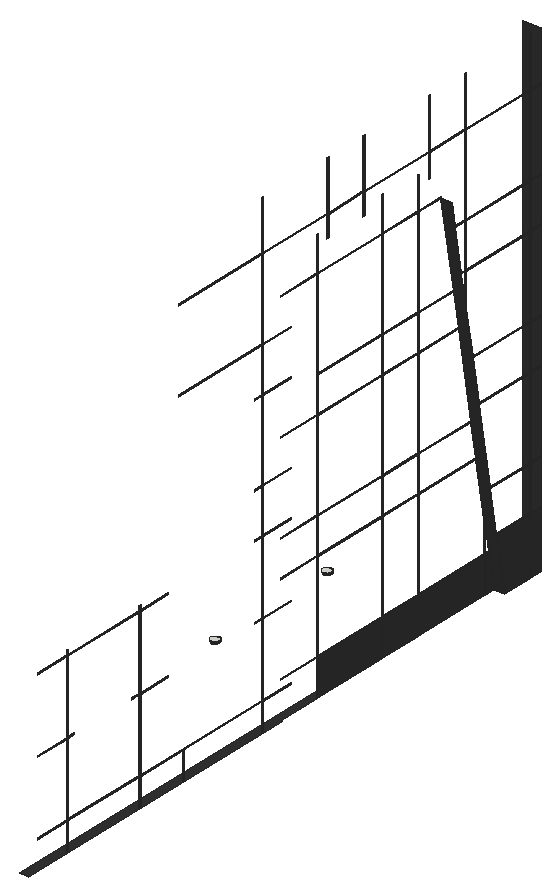
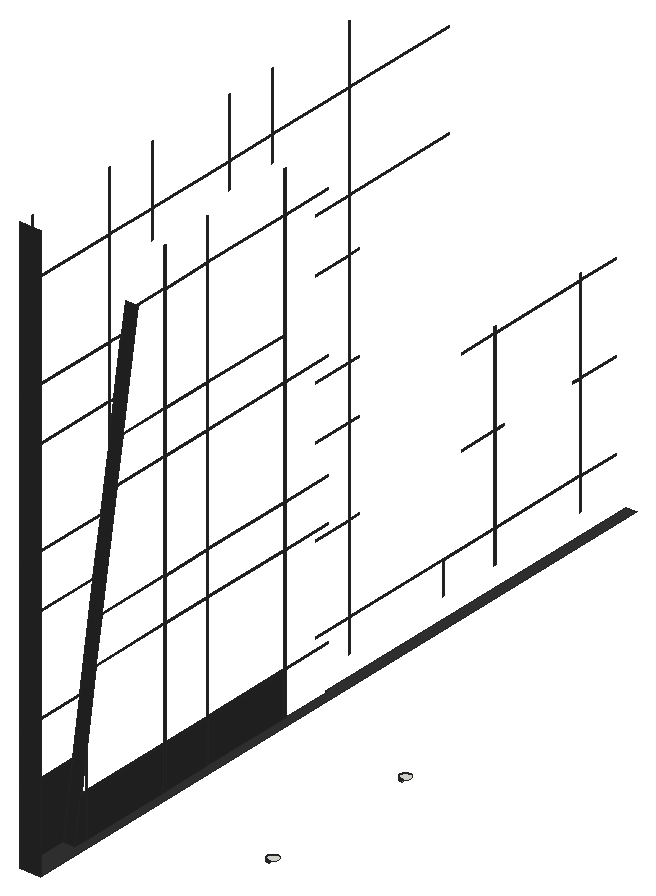
# SketchUp Ruby script. Lengths in inches.
U = 1.inch
M = Sketchup.active_model
def pt(a) = Geom::Point3d.new(a.map { |v| v * U })
def face(e, loops, mat)
  f = e.add_face(loops[0].map { |a| pt(a) })
  loops[1..].each { |l| e.add_face(l.map { |a| pt(a) }).erase! }
  f.material = f.back_material = mat if mat
  f
end
# faces: each face lists its corners as indices into pts; further lists are holes
def faces(e, pts, list, mat = nil) = list.each { |f| face(e, (f[0].is_a?(Array) ? f : [f]).map { |l| l.map { |i| pts[i] } }, mat) }
# xy, xz, yz: faces in a plane at the given z, y or x. An outline is a flat list of corners, or four numbers for a rectangle; further outlines are holes
def ring(l) = l.size == 4 ? [[l[0], l[1]], [l[2], l[1]], [l[2], l[3]], [l[0], l[3]]] : l.each_slice(2).to_a
def flat(e, list, mat, &to3) = list.each { |f| face(e, (f[0].is_a?(Array) ? f : [f]).map { |l| ring(l).map { |u, v| to3.(u, v) } }, mat) }
def xy(e, z, list, mat = nil) = flat(e, list, mat) { |x, y| [x, y, z] }
def xz(e, y, list, mat = nil) = flat(e, list, mat) { |x, z| [x, y, z] }
def yz(e, x, list, mat = nil) = flat(e, list, mat) { |y, z| [x, y, z] }
def lines(e, pts, list) = list.each { |a, b| e.add_line(pt(pts[a]), pt(pts[b])) }
# prism: a flat outline (further loops are holes) pulled along v
def prism(e, loops, v, mat = nil)
  f = face(e, loops, mat); d = Geom::Vector3d.new(v.map { |x| x * U })
  f.pushpull(f.normal.samedirection?(d) ? d.length : -d.length)
end
def box(e, o, s, mat = nil) = prism(e, [[o, [o[0] + s[0], o[1], o[2]], [o[0] + s[0], o[1] + s[1], o[2]], [o[0], o[1] + s[1], o[2]]]], [0, 0, s[2]], mat)
def at(x, y, z, deg = 0) = Geom::Transformation.translation(pt([x, y, z])) * Geom::Transformation.rotation(ORIGIN, Z_AXIS, deg.degrees)
def axes(o, x, y, z) = Geom::Transformation.new([*x, 0, *y, 0, *z, 0, *pt(o).to_a, 1])
def part(name) = M.definitions.add(name)
# library, detail: a bought-in or finely detailed component or shape, given as its bounding box
def library(name, o, s) = part(name).tap { |d| box(d.entities, o, s) }
def detail(e, o, s) = box(e.add_group.entities, o, s)
def put(e, d, t, mat = nil) = e.add_instance(d, t).tap { |i| i.material = mat if mat }
def group(e, t, mat = nil) = e.add_group.tap { |g| g.transformation = t; g.material = mat if mat }.entities
root = M.entities
M.materials.add("[Granite Dark Gray]").color = [51, 50, 50]
xy(root,126,[[432,183,432,600,444,600,444,592,443.875,592,443.875,591,444,591,444,570,437,570,437,563,436.875,563,436.875,562,437,562,437,508,436.875,508,436.875,507,437,507,437,478,436.875,478,436.875,477,437,477,437,424,436.875,424,436.875,423,437,423,437,393,438,393,438,183]],"[Granite Dark Gray]")
xy(root,129,[[359.84,432,359.76,432.01,359.6875,432.02,359.61,432.03,359.45,432.05,359.375,432.07,359.3,432.08,359.22,432.1,359.15,432.125,359.07,432.15,359,432.17,358.92,432.2,358.71,432.29,358.64,432.33,358.57,432.36,358.43,432.44,358.37,432.48,358.3,432.53,358.24,432.57,358.17,432.62,357.93,432.82,357.88,432.88,357.82,432.93,357.62,433.17,357.57,433.24,357.53,433.3,357.48,433.37,357.44,433.43,357.36,433.57,357.33,433.64,357.29,433.71,357.2,433.92,357.17,434,357.15,434.07,357.125,434.15,357.1,434.22,357.08,434.3,357.07,434.375,357.05,434.45,357.03,434.61,357.02,434.6875,357.01,434.76,357,434.84,357,435.16,357.01,435.24,357.02,435.3125,357.03,435.39,357.05,435.55,357.07,435.625,357.08,435.7,357.1,435.78,357.125,435.85,357.15,435.93,357.17,436,357.2,436.08,357.29,436.29,357.33,436.36,357.36,436.43,357.44,436.57,357.48,436.63,357.53,436.7,357.57,436.76,357.62,436.83,357.82,437.07,357.88,437.12,357.93,437.18,358.17,437.38,358.24,437.43,358.3,437.47,358.37,437.52,358.43,437.56,358.57,437.64,358.64,437.67,358.71,437.71,358.92,437.8,359,437.83,359.07,437.85,359.15,437.875,359.22,437.9,359.3,437.92,359.375,437.93,359.45,437.95,359.61,437.97,359.6875,437.98,359.76,437.99,359.84,438,360.16,438,360.24,437.99,360.3125,437.98,360.39,437.97,360.55,437.95,360.625,437.93,360.7,437.92,360.78,437.9,360.85,437.875,360.93,437.85,361,437.83,361.08,437.8,361.29,437.71,361.36,437.67,361.43,437.64,361.57,437.56,361.63,437.52,361.7,437.47,361.76,437.43,361.83,437.38,362.07,437.18,362.12,437.12,362.18,437.07,362.38,436.83,362.43,436.76,362.47,436.7,362.52,436.63,362.56,436.57,362.64,436.43,362.67,436.36,362.71,436.29,362.8,436.08,362.83,436,362.85,435.93,362.875,435.85,362.9,435.78,362.92,435.7,362.93,435.625,362.95,435.55,362.97,435.39,362.98,435.3125,362.99,435.24,363,435.16,363,434.84,362.99,434.76,362.98,434.6875,362.97,434.61,362.95,434.45,362.93,434.375,362.92,434.3,362.9,434.22,362.875,434.15,362.85,434.07,362.83,434,362.8,433.92,362.71,433.71,362.67,433.64,362.64,433.57,362.56,433.43,362.52,433.37,362.47,433.3,362.43,433.24,362.38,433.17,362.18,432.93,362.12,432.88,362.07,432.82,361.83,432.62,361.76,432.57,361.7,432.53,361.63,432.48,361.57,432.44,361.43,432.36,361.36,432.33,361.29,432.29,361.08,432.2,361,432.17,360.93,432.15,360.85,432.125,360.78,432.1,360.7,432.08,360.625,432.07,360.55,432.05,360.39,432.03,360.3125,432.02,360.24,432.01,360.16,432],[359.84,525,359.76,525.01,359.6875,525.02,359.61,525.03,359.45,525.05,359.375,525.07,359.3,525.08,359.22,525.1,359.15,525.125,359.07,525.15,359,525.17,358.92,525.2,358.71,525.29,358.64,525.33,358.57,525.36,358.43,525.44,358.37,525.48,358.3,525.53,358.24,525.57,358.17,525.62,357.93,525.82,357.88,525.88,357.82,525.93,357.62,526.17,357.57,526.24,357.53,526.3,357.48,526.37,357.44,526.43,357.36,526.57,357.33,526.64,357.29,526.71,357.2,526.92,357.17,527,357.15,527.07,357.125,527.15,357.1,527.22,357.08,527.3,357.07,527.375,357.05,527.45,357.03,527.61,357.02,527.6875,357.01,527.76,357,527.84,357,528.16,357.01,528.24,357.02,528.3125,357.03,528.39,357.05,528.55,357.07,528.625,357.08,528.7,357.1,528.78,357.125,528.85,357.15,528.93,357.17,529,357.2,529.08,357.29,529.29,357.33,529.36,357.36,529.43,357.44,529.57,357.48,529.63,357.53,529.7,357.57,529.76,357.62,529.83,357.82,530.07,357.88,530.12,357.93,530.18,358.17,530.38,358.24,530.43,358.3,530.47,358.37,530.52,358.43,530.56,358.57,530.64,358.64,530.67,358.71,530.71,358.92,530.8,359,530.83,359.07,530.85,359.15,530.875,359.22,530.9,359.3,530.92,359.375,530.93,359.45,530.95,359.61,530.97,359.6875,530.98,359.76,530.99,359.84,531,360.16,531,360.24,530.99,360.3125,530.98,360.39,530.97,360.55,530.95,360.625,530.93,360.7,530.92,360.78,530.9,360.85,530.875,360.93,530.85,361,530.83,361.08,530.8,361.29,530.71,361.36,530.67,361.43,530.64,361.57,530.56,361.63,530.52,361.7,530.47,361.76,530.43,361.83,530.38,362.07,530.18,362.12,530.12,362.18,530.07,362.38,529.83,362.43,529.76,362.47,529.7,362.52,529.63,362.56,529.57,362.64,529.43,362.67,529.36,362.71,529.29,362.8,529.08,362.83,529,362.85,528.93,362.875,528.85,362.9,528.78,362.92,528.7,362.93,528.625,362.95,528.55,362.97,528.39,362.98,528.3125,362.99,528.24,363,528.16,363,527.84,362.99,527.76,362.98,527.6875,362.97,527.61,362.95,527.45,362.93,527.375,362.92,527.3,362.9,527.22,362.875,527.15,362.85,527.07,362.83,527,362.8,526.92,362.71,526.71,362.67,526.64,362.64,526.57,362.56,526.43,362.52,526.37,362.47,526.3,362.43,526.24,362.38,526.17,362.18,525.93,362.12,525.88,362.07,525.82,361.83,525.62,361.76,525.57,361.7,525.53,361.63,525.48,361.57,525.44,361.43,525.36,361.36,525.33,361.29,525.29,361.08,525.2,361,525.17,360.93,525.15,360.85,525.125,360.78,525.1,360.7,525.08,360.625,525.07,360.55,525.05,360.39,525.03,360.3125,525.02,360.24,525.01,360.16,525]])
xz(root,423,[[436.875,126,437,150]],"[Granite Dark Gray]")
xz(root,424,[[436.875,126,437,150]],"[Granite Dark Gray]")
xz(root,432,[[359.84,128,359.92,129],[359.92,128,360,129],[360,128,360.08,129],[360.08,128,360.16,129]])
xz(root,438,[[359.84,128,359.92,129],[359.92,128,360,129],[360,128,360.08,129],[360.08,128,360.16,129]])
xz(root,477,[[436.875,126,437,150]],"[Granite Dark Gray]")
xz(root,478,[[436.875,126,437,150]],"[Granite Dark Gray]")
xz(root,507,[[436.875,126,437,150]],"[Granite Dark Gray]")
xz(root,508,[[436.875,126,437,150]],"[Granite Dark Gray]")
xz(root,525,[[359.84,128,359.92,129],[359.92,128,360,129],[360,128,360.08,129],[360.08,128,360.16,129]])
xz(root,531,[[359.84,128,359.92,129],[359.92,128,360,129],[360,128,360.08,129],[360.08,128,360.16,129]])
xz(root,562,[[436.875,126,437,150]],"[Granite Dark Gray]")
xz(root,563,[[436.875,126,437,150]],"[Granite Dark Gray]")
xz(root,591,[[443.875,126,444,150]],"[Granite Dark Gray]")
xz(root,592,[[443.875,126,444,150]],"[Granite Dark Gray]")
xz(root,600,[[432,126,432,450,444,450,444,417,443.875,417,443.875,416,444,416,444,363,443.875,363,443.875,362,444,362,444,333,443.875,333,443.875,332,444,332,444,279,443.875,279,443.875,278,444,278,444,249,443.875,249,443.875,248,444,248,444,195,443.875,195,443.875,194,444,194,444,165,443.875,165,443.875,164,444,164,444,126]],"[Granite Dark Gray]")
yz(root,363,[[434.84,128,434.92,129],[434.92,128,435,129],[435,128,435.08,129],[435.08,128,435.16,129],[527.84,128,527.92,129],
  [527.92,128,528,129],[528,128,528.08,129],[528.08,128,528.16,129]])
yz(root,436.875,[[[423,126,424,126,424,150,477,150,477,126,478,126,478,150,507,150,507,126,508,126,508,150,562,150,562,126,563,126,563,150,565.83,150,565.65,151,563,151,563,166.25,562,172,562,151,508,151,508,210,555.39,210,555.22,211,508,211,508,234,551.22,234,551.04,235,508,235,508,294,540.78,294,540.61,295,508,295,508,318,536.61,318,536.43,319,508,319,508,378,526.17,378,526.11,378.35,526.07,378.62,526.02,378.88,525.99,379,508,379,508,400.19,507.9,400.23,507.4,400.41,507.15,400.49,507,400.54,507,379,478,379,478,402,477,402,477,379,424,379,424,402,423,402,423,379,393,379,393,378,423,378,423,319,424,319,424,378,477,378,477,319,423,319,423,318,477,318,477,295,424,295,424,318,423,318,423,295,393,295,393,294,423,294,423,235,393,235,393,234,423,234,423,211,393,211,393,210,423,210,423,151,393,151,393,150,423,150],[424,235,477,294],[424,151,477,210],[478,319,507,378],[478,151,507,210],[478,235,507,294],[424,211,477,234],[478,211,507,234],[478,295,507,318]]],"[Granite Dark Gray]")
yz(root,437,[[424,126,477,150],[478,126,507,150],[508,126,562,150],[563,126,570,126,565.83,150,563,150]],"[Granite Dark Gray]")
yz(root,443.875,[[[591,126,592,126,592,164,600,164,600,165,592,165,592,194,600,194,600,195,592,195,592,248,600,248,600,249,592,249,592,278,600,278,600,279,592,279,592,332,600,332,600,333,592,333,592,362,600,362,600,363,592,363,592,416,600,416,600,417,592,417,592,450,591,450,591,417,538,417,538,450,537,450,537,417,508,417,508,450,507,450,507,417,454,417,454,450,453,450,453,417,424,417,424,450,423,450,423,417,370,417,370,450,369,450,369,417,300,417,300,416,369,416,369,363,300,363,300,362,369,362,369,333,363,333,363,332,369,332,369,279,363,279,363,278,369,278,369,249,363,249,363,248,369,248,369,200,363,200,363,199,369,199,369,151,268,151,268,199,291,199,291,200,268,200,268,248,291,248,291,249,268,249,268,252,267,252,267,249,208,249,208,252,207,252,207,249,183,249,183,248,207,248,207,200,183,200,183,199,207,199,207,151,183,151,183,150,207,150,207,132,208,132,208,150,267,150,267,132,268,132,268,150,303,150,303,132,304,132,304,150,369,150,369,132,370,132,370,150,393,150,393,151,370,151,370,199,393,199,393,200,370,200,370,248,393,248,393,249,370,249,370,278,393,278,393,279,370,279,370,332,393,332,393,333,370,333,370,362,393,362,393,363,370,363,370,416,423,416,423,402,424,402,424,416,453,416,453,402,454,402,454,416,507,416,507,400.54,507.15,400.49,507.4,400.41,507.9,400.23,508,400.19,508,416,537,416,537,363,528.78,363,528.96,362,537,362,537,333,534,333,534.17,332,537,332,537,315.75,538,310,538,332,591,332,591,279,543.39,279,543.57,278,591,278,591,249,548.61,249,548.78,248,591,248,591,195,558,195,558.17,194,591,194,591,165,563.22,165,563.39,164,591,164],[208,151,208,199,213,199,213,200,208,200,208,248,267,248,267,200,261,200,261,199,267,199,267,151],[538,363,591,416],[538,333,591,362]]],"[Granite Dark Gray]")
yz(root,444,[[570,126,591,126,591,164,563.39,164],[592,126,600,164]],"[Granite Dark Gray]")
p = [[444,528.78,363],[444,526.11,378.35],[436.875,526.11,378.35],[436.875,526.17,378],[437,526.17,378],[437,536.43,319],
  [436.875,536.43,319],[436.875,536.61,318],[437,536.61,318],[437,540.61,295],[436.875,540.61,295],[436.875,540.78,294],
  [437,540.78,294],[437,551.04,235],[436.875,551.04,235],[436.875,551.22,234],[437,551.22,234],[437,555.22,211],
  [436.875,555.22,211],[436.875,555.39,210],[437,555.39,210],[437,562,172],[436.875,562,172],[436.875,563,166.25],
  [437,563,166.25],[437,565.65,151],[436.875,565.65,151],[436.875,565.83,150],[437,565.83,150],[437,570,126],
  [444,570,126],[444,563.39,164],[443.875,563.39,164],[443.875,563.22,165],[444,563.22,165],[444,558.17,194],
  [443.875,558.17,194],[443.875,558,195],[444,558,195],[444,548.78,248],[443.875,548.78,248],[443.875,548.61,249],
  [444,548.61,249],[444,543.57,278],[443.875,543.57,278],[443.875,543.39,279],[444,543.39,279],[444,538,310],
  [443.875,538,310],[443.875,537,315.75],[444,537,315.75],[444,534.17,332],[443.875,534.17,332],[443.875,534,333],
  [444,534,333],[444,528.96,362],[443.875,528.96,362],[443.875,528.78,363],[359.61,432.03,128],[359.53,432.04,128],
  [359.53,432.04,129],[359.61,432.03,129],[359.45,432.05,128],[359.45,432.05,129],[359.6875,432.02,128],[359.6875,432.02,129],
  [359.76,432.01,128],[359.76,432.01,129],[359.84,432,128],[359.84,432,129],[360.24,432.01,128],[360.16,432,128],
  [360.16,432,129],[360.24,432.01,129],[360.3125,432.02,128],[360.3125,432.02,129],[360.39,432.03,128],[360.39,432.03,129],
  [360.47,432.04,128],[360.47,432.04,129],[360.55,432.05,128],[360.55,432.05,129],[359.375,432.07,128],[359.3,432.08,128],
  [359.3,432.08,129],[359.375,432.07,129],[360.625,432.07,128],[360.625,432.07,129],[360.7,432.08,128],[360.7,432.08,129],
  [360.78,432.1,128],[360.78,432.1,129],[360.85,432.125,128],[360.85,432.125,129],[360.93,432.15,128],[360.93,432.15,129],
  [361,432.17,128],[361,432.17,129],[361.08,432.2,128],[361.08,432.2,129],[361.15,432.23,128],[361.15,432.23,129],
  [361.22,432.26,128],[361.22,432.26,129],[361.29,432.29,128],[361.29,432.29,129],[361.36,432.33,128],[361.36,432.33,129],
  [361.43,432.36,128],[361.43,432.36,129],[361.5,432.4,128],[361.5,432.4,129],[361.57,432.44,128],[361.57,432.44,129],
  [361.63,432.48,128],[361.63,432.48,129],[361.7,432.53,128],[361.7,432.53,129],[361.76,432.57,128],[361.76,432.57,129],
  [361.83,432.62,128],[361.83,432.62,129],[361.89,432.67,128],[361.89,432.67,129],[361.95,432.72,128],[361.95,432.72,129],
  [362.01,432.77,128],[362.01,432.77,129],[362.07,432.82,128],[362.07,432.82,129],[362.12,432.88,128],[362.12,432.88,129],
  [362.18,432.93,128],[362.18,432.93,129],[362.23,432.99,128],[362.23,432.99,129],[362.28,433.05,128],[362.28,433.05,129],
  [362.33,433.11,128],[362.33,433.11,129],[362.38,433.17,128],[362.38,433.17,129],[362.43,433.24,128],[362.43,433.24,129],
  [362.47,433.3,128],[362.47,433.3,129],[362.52,433.37,128],[362.52,433.37,129],[362.56,433.43,128],[362.56,433.43,129],
  [362.6,433.5,128],[362.6,433.5,129],[362.64,433.57,128],[362.64,433.57,129],[362.67,433.64,128],[362.67,433.64,129],
  [362.71,433.71,128],[362.71,433.71,129],[362.74,433.78,128],[362.74,433.78,129],[362.77,433.85,128],[362.77,433.85,129],
  [362.8,433.92,128],[362.8,433.92,129],[362.83,434,128],[362.83,434,129],[362.85,434.07,128],[362.85,434.07,129],
  [362.875,434.15,128],[362.875,434.15,129],[362.9,434.22,128],[362.9,434.22,129],[362.92,434.3,128],[362.92,434.3,129],
  [362.93,434.375,128],[362.93,434.375,129],[362.95,434.45,128],[362.95,434.45,129],[362.96,434.53,128],[362.96,434.53,129],
  [362.97,434.61,128],[362.97,434.61,129],[362.98,434.6875,128],[362.98,434.6875,129],[362.99,434.76,128],[362.99,434.76,129],
  [363,434.84,128],[363,434.84,129],[362.99,435.24,128],[363,435.16,128],[363,435.16,129],[362.99,435.24,129],
  [362.98,435.3125,128],[362.98,435.3125,129],[362.97,435.39,128],[362.97,435.39,129],[362.96,435.47,128],[362.96,435.47,129],
  [362.95,435.55,128],[362.95,435.55,129],[362.93,435.625,128],[362.93,435.625,129],[362.92,435.7,128],[362.92,435.7,129],
  [362.9,435.78,128],[362.9,435.78,129],[362.875,435.85,128],[362.875,435.85,129],[362.83,436,128],[362.85,435.93,128],
  [362.85,435.93,129],[362.83,436,129],[362.8,436.08,128],[362.8,436.08,129],[362.74,436.22,128],[362.77,436.15,128],
  [362.77,436.15,129],[362.74,436.22,129],[362.71,436.29,128],[362.71,436.29,129],[362.67,436.36,128],[362.67,436.36,129],
  [362.64,436.43,128],[362.64,436.43,129],[362.6,436.5,128],[362.6,436.5,129],[362.56,436.57,128],[362.56,436.57,129],
  [362.52,436.63,128],[362.52,436.63,129],[362.47,436.7,128],[362.47,436.7,129],[362.43,436.76,128],[362.43,436.76,129],
  [362.33,436.89,128],[362.38,436.83,128],[362.38,436.83,129],[362.33,436.89,129],[362.23,437.01,128],[362.28,436.95,128],
  [362.28,436.95,129],[362.23,437.01,129],[362.18,437.07,128],[362.18,437.07,129],[362.12,437.12,128],[362.12,437.12,129],
  [362.07,437.18,128],[362.07,437.18,129],[361.95,437.28,128],[362.01,437.23,128],[362.01,437.23,129],[361.95,437.28,129],
  [361.83,437.38,128],[361.89,437.33,128],[361.89,437.33,129],[361.83,437.38,129],[361.7,437.47,128],[361.76,437.43,128],
  [361.76,437.43,129],[361.7,437.47,129],[361.63,437.52,128],[361.63,437.52,129],[361.57,437.56,128],[361.57,437.56,129],
  [361.43,437.64,128],[361.5,437.6,128],[361.5,437.6,129],[361.43,437.64,129],[361.36,437.67,128],[361.36,437.67,129],
  [361.15,437.77,128],[361.22,437.74,128],[361.22,437.74,129],[361.15,437.77,129],[361.29,437.71,128],[361.29,437.71,129],
  [360.93,437.85,128],[361,437.83,128],[361,437.83,129],[360.93,437.85,129],[361.08,437.8,128],[361.08,437.8,129],
  [359.3,437.92,128],[359.375,437.93,128],[359.375,437.93,129],[359.3,437.92,129],[359.45,437.95,128],[359.45,437.95,129],
  [359.53,437.96,128],[359.53,437.96,129],[360.55,437.95,128],[360.625,437.93,128],[360.625,437.93,129],[360.55,437.95,129],
  [360.47,437.96,128],[360.47,437.96,129],[360.7,437.92,128],[360.7,437.92,129],[360.78,437.9,128],[360.78,437.9,129],
  [360.85,437.875,128],[360.85,437.875,129],[359.61,437.97,128],[359.61,437.97,129],[359.6875,437.98,128],[359.6875,437.98,129],
  [359.76,437.99,128],[359.76,437.99,129],[359.84,438,128],[359.84,438,129],[360.24,437.99,128],[360.3125,437.98,128],
  [360.3125,437.98,129],[360.24,437.99,129],[360.16,438,128],[360.16,438,129],[360.39,437.97,128],[360.39,437.97,129],
  [359.61,525.03,128],[359.53,525.04,128],[359.53,525.04,129],[359.61,525.03,129],[359.45,525.05,128],[359.45,525.05,129],
  [359.6875,525.02,128],[359.6875,525.02,129],[359.76,525.01,128],[359.76,525.01,129],[359.84,525,128],[359.84,525,129],
  [360.24,525.01,128],[360.16,525,128],[360.16,525,129],[360.24,525.01,129],[360.3125,525.02,128],[360.3125,525.02,129],
  [360.39,525.03,128],[360.39,525.03,129],[360.47,525.04,128],[360.47,525.04,129],[360.55,525.05,128],[360.55,525.05,129],
  [359.375,525.07,128],[359.3,525.08,128],[359.3,525.08,129],[359.375,525.07,129],[360.625,525.07,128],[360.625,525.07,129],
  [360.7,525.08,128],[360.7,525.08,129],[360.78,525.1,128],[360.78,525.1,129],[360.85,525.125,128],[360.85,525.125,129],
  [360.93,525.15,128],[360.93,525.15,129],[361,525.17,128],[361,525.17,129],[361.08,525.2,128],[361.08,525.2,129],
  [361.15,525.23,128],[361.15,525.23,129],[361.22,525.26,128],[361.22,525.26,129],[361.29,525.29,128],[361.29,525.29,129],
  [361.36,525.33,128],[361.36,525.33,129],[361.43,525.36,128],[361.43,525.36,129],[361.5,525.4,128],[361.5,525.4,129],
  [361.57,525.44,128],[361.57,525.44,129],[361.63,525.48,128],[361.63,525.48,129],[361.7,525.53,128],[361.7,525.53,129],
  [361.76,525.57,128],[361.76,525.57,129],[361.83,525.62,128],[361.83,525.62,129],[361.89,525.67,128],[361.89,525.67,129],
  [361.95,525.72,128],[361.95,525.72,129],[362.01,525.77,128],[362.01,525.77,129],[362.07,525.82,128],[362.07,525.82,129],
  [362.12,525.88,128],[362.12,525.88,129],[362.18,525.93,128],[362.18,525.93,129],[362.23,525.99,128],[362.23,525.99,129],
  [362.28,526.05,128],[362.28,526.05,129],[362.33,526.11,128],[362.33,526.11,129],[362.38,526.17,128],[362.38,526.17,129],
  [362.43,526.24,128],[362.43,526.24,129],[362.47,526.3,128],[362.47,526.3,129],[362.52,526.37,128],[362.52,526.37,129],
  [362.56,526.43,128],[362.56,526.43,129],[362.6,526.5,128],[362.6,526.5,129],[362.64,526.57,128],[362.64,526.57,129],
  [362.67,526.64,128],[362.67,526.64,129],[362.71,526.71,128],[362.71,526.71,129],[362.74,526.78,128],[362.74,526.78,129],
  [362.77,526.85,128],[362.77,526.85,129],[362.8,526.92,128],[362.8,526.92,129],[362.83,527,128],[362.83,527,129],
  [362.85,527.07,128],[362.85,527.07,129],[362.875,527.15,128],[362.875,527.15,129],[362.9,527.22,128],[362.9,527.22,129],
  [362.92,527.3,128],[362.92,527.3,129],[362.93,527.375,128],[362.93,527.375,129],[362.95,527.45,128],[362.95,527.45,129],
  [362.96,527.53,128],[362.96,527.53,129],[362.97,527.61,128],[362.97,527.61,129],[362.98,527.6875,128],[362.98,527.6875,129],
  [362.99,527.76,128],[362.99,527.76,129],[363,527.84,128],[363,527.84,129],[362.99,528.24,128],[363,528.16,128],
  [363,528.16,129],[362.99,528.24,129],[362.98,528.3125,128],[362.98,528.3125,129],[362.97,528.39,128],[362.97,528.39,129],
  [362.96,528.47,128],[362.96,528.47,129],[362.95,528.55,128],[362.95,528.55,129],[362.93,528.625,128],[362.93,528.625,129],
  [362.92,528.7,128],[362.92,528.7,129],[362.9,528.78,128],[362.9,528.78,129],[362.875,528.85,128],[362.875,528.85,129],
  [362.83,529,128],[362.85,528.93,128],[362.85,528.93,129],[362.83,529,129],[362.8,529.08,128],[362.8,529.08,129],
  [362.74,529.22,128],[362.77,529.15,128],[362.77,529.15,129],[362.74,529.22,129],[362.71,529.29,128],[362.71,529.29,129],
  [362.67,529.36,128],[362.67,529.36,129],[362.64,529.43,128],[362.64,529.43,129],[362.6,529.5,128],[362.6,529.5,129],
  [362.56,529.57,128],[362.56,529.57,129],[362.52,529.63,128],[362.52,529.63,129],[362.47,529.7,128],[362.47,529.7,129],
  [362.43,529.76,128],[362.43,529.76,129],[362.33,529.89,128],[362.38,529.83,128],[362.38,529.83,129],[362.33,529.89,129],
  [362.23,530.01,128],[362.28,529.95,128],[362.28,529.95,129],[362.23,530.01,129],[362.18,530.07,128],[362.18,530.07,129],
  [362.12,530.12,128],[362.12,530.12,129],[362.07,530.18,128],[362.07,530.18,129],[361.95,530.28,128],[362.01,530.23,128],
  [362.01,530.23,129],[361.95,530.28,129],[361.83,530.38,128],[361.89,530.33,128],[361.89,530.33,129],[361.83,530.38,129],
  [361.7,530.47,128],[361.76,530.43,128],[361.76,530.43,129],[361.7,530.47,129],[361.63,530.52,128],[361.63,530.52,129],
  [361.57,530.56,128],[361.57,530.56,129],[361.43,530.64,128],[361.5,530.6,128],[361.5,530.6,129],[361.43,530.64,129],
  [361.36,530.67,128],[361.36,530.67,129],[361.15,530.77,128],[361.22,530.74,128],[361.22,530.74,129],[361.15,530.77,129],
  [361.29,530.71,128],[361.29,530.71,129],[360.93,530.85,128],[361,530.83,128],[361,530.83,129],[360.93,530.85,129],
  [361.08,530.8,128],[361.08,530.8,129],[359.3,530.92,128],[359.375,530.93,128],[359.375,530.93,129],[359.3,530.92,129],
  [359.45,530.95,128],[359.45,530.95,129],[359.53,530.96,128],[359.53,530.96,129],[360.55,530.95,128],[360.625,530.93,128],
  [360.625,530.93,129],[360.55,530.95,129],[360.47,530.96,128],[360.47,530.96,129],[360.7,530.92,128],[360.7,530.92,129],
  [360.78,530.9,128],[360.78,530.9,129],[360.85,530.875,128],[360.85,530.875,129],[359.61,530.97,128],[359.61,530.97,129],
  [359.6875,530.98,128],[359.6875,530.98,129],[359.76,530.99,128],[359.76,530.99,129],[359.84,531,128],[359.84,531,129],
  [360.24,530.99,128],[360.3125,530.98,128],[360.3125,530.98,129],[360.24,530.99,129],[360.16,531,128],[360.16,531,129],
  [360.39,530.97,128],[360.39,530.97,129]]
faces(root,p,[[0,1,2,3,4,5,6,7,8,9,10,11,12,13,14,15,16,17,18,19,20,21,22,23,24,25,26,27,28,29,30,31,32,33,34,35,36,37,38,39,40,41,42,43,44,45,46,47,48,49,50,51,52,53,54,55,56,57]],"[Granite Dark Gray]")
faces(root,p,[[58,59,60,61],[59,62,63,60],[64,58,61,65],[66,64,65,67],[68,66,67,69],[70,71,72,73],[74,70,73,75],[76,74,75,77],
  [78,76,77,79],[80,78,79,81],[82,83,84,85],[62,82,85,63],[86,80,81,87],[88,86,87,89],[90,88,89,91],[92,90,91,93],
  [94,92,93,95],[96,94,95,97],[98,96,97,99],[100,98,99,101],[102,100,101,103],[104,102,103,105],[106,104,105,107],[108,106,107,109],
  [110,108,109,111],[112,110,111,113],[114,112,113,115],[116,114,115,117],[118,116,117,119],[120,118,119,121],[122,120,121,123],[124,122,123,125],
  [126,124,125,127],[128,126,127,129],[130,128,129,131],[132,130,131,133],[134,132,133,135],[136,134,135,137],[138,136,137,139],[140,138,139,141],
  [142,140,141,143],[144,142,143,145],[146,144,145,147],[148,146,147,149],[150,148,149,151],[152,150,151,153],[154,152,153,155],[156,154,155,157],
  [158,156,157,159],[160,158,159,161],[162,160,161,163],[164,162,163,165],[166,164,165,167],[168,166,167,169],[170,168,169,171],[172,170,171,173],
  [174,172,173,175],[176,174,175,177],[178,176,177,179],[180,178,179,181],[182,180,181,183],[184,182,183,185],[186,184,185,187],[188,189,190,191],
  [192,188,191,193],[194,192,193,195],[196,194,195,197],[198,196,197,199],[200,198,199,201],[202,200,201,203],[204,202,203,205],[206,204,205,207],
  [208,209,210,211],[209,206,207,210],[212,208,211,213],[214,215,216,217],[215,212,213,216],[218,214,217,219],[220,218,219,221],[222,220,221,223],
  [224,222,223,225],[226,224,225,227],[228,226,227,229],[230,228,229,231],[232,230,231,233],[234,235,236,237],[235,232,233,236],[238,239,240,241],
  [239,234,237,240],[242,238,241,243],[244,242,243,245],[246,244,245,247],[248,249,250,251],[249,246,247,250],[252,253,254,255],[253,248,251,254],
  [256,257,258,259],[257,252,255,258],[260,256,259,261],[262,260,261,263],[264,265,266,267],[268,264,267,269],[265,262,263,266],[270,271,272,273],
  [271,274,275,272],[274,268,269,275],[276,277,278,279],[277,280,281,278],[280,270,273,281],[282,283,284,285],[283,286,287,284],[286,288,289,287],
  [290,291,292,293],[294,290,293,295],[291,296,297,292],[296,298,299,297],[298,300,301,299],[300,276,279,301],[288,302,303,289],[302,304,305,303],
  [304,306,307,305],[306,308,309,307],[310,311,312,313],[314,310,313,315],[311,316,317,312],[316,294,295,317],[318,319,320,321],[319,322,323,320],
  [324,318,321,325],[326,324,325,327],[328,326,327,329],[330,331,332,333],[334,330,333,335],[336,334,335,337],[338,336,337,339],[340,338,339,341],
  [342,343,344,345],[322,342,345,323],[346,340,341,347],[348,346,347,349],[350,348,349,351],[352,350,351,353],[354,352,353,355],[356,354,355,357],
  [358,356,357,359],[360,358,359,361],[362,360,361,363],[364,362,363,365],[366,364,365,367],[368,366,367,369],[370,368,369,371],[372,370,371,373],
  [374,372,373,375],[376,374,375,377],[378,376,377,379],[380,378,379,381],[382,380,381,383],[384,382,383,385],[386,384,385,387],[388,386,387,389],
  [390,388,389,391],[392,390,391,393],[394,392,393,395],[396,394,395,397],[398,396,397,399],[400,398,399,401],[402,400,401,403],[404,402,403,405],
  [406,404,405,407],[408,406,407,409],[410,408,409,411],[412,410,411,413],[414,412,413,415],[416,414,415,417],[418,416,417,419],[420,418,419,421],
  [422,420,421,423],[424,422,423,425],[426,424,425,427],[428,426,427,429],[430,428,429,431],[432,430,431,433],[434,432,433,435],[436,434,435,437],
  [438,436,437,439],[440,438,439,441],[442,440,441,443],[444,442,443,445],[446,444,445,447],[448,449,450,451],[452,448,451,453],[454,452,453,455],
  [456,454,455,457],[458,456,457,459],[460,458,459,461],[462,460,461,463],[464,462,463,465],[466,464,465,467],[468,469,470,471],[469,466,467,470],
  [472,468,471,473],[474,475,476,477],[475,472,473,476],[478,474,477,479],[480,478,479,481],[482,480,481,483],[484,482,483,485],[486,484,485,487],
  [488,486,487,489],[490,488,489,491],[492,490,491,493],[494,495,496,497],[495,492,493,496],[498,499,500,501],[499,494,497,500],[502,498,501,503],
  [504,502,503,505],[506,504,505,507],[508,509,510,511],[509,506,507,510],[512,513,514,515],[513,508,511,514],[516,517,518,519],[517,512,515,518],
  [520,516,519,521],[522,520,521,523],[524,525,526,527],[528,524,527,529],[525,522,523,526],[530,531,532,533],[531,534,535,532],[534,528,529,535],
  [536,537,538,539],[537,540,541,538],[540,530,533,541],[542,543,544,545],[543,546,547,544],[546,548,549,547],[550,551,552,553],[554,550,553,555],
  [551,556,557,552],[556,558,559,557],[558,560,561,559],[560,536,539,561],[548,562,563,549],[562,564,565,563],[564,566,567,565],[566,568,569,567],
  [570,571,572,573],[574,570,573,575],[571,576,577,572],[576,554,555,577]])
